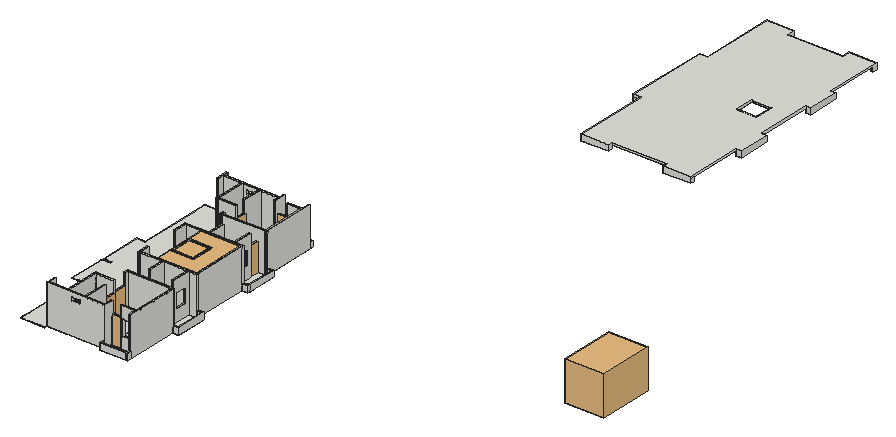
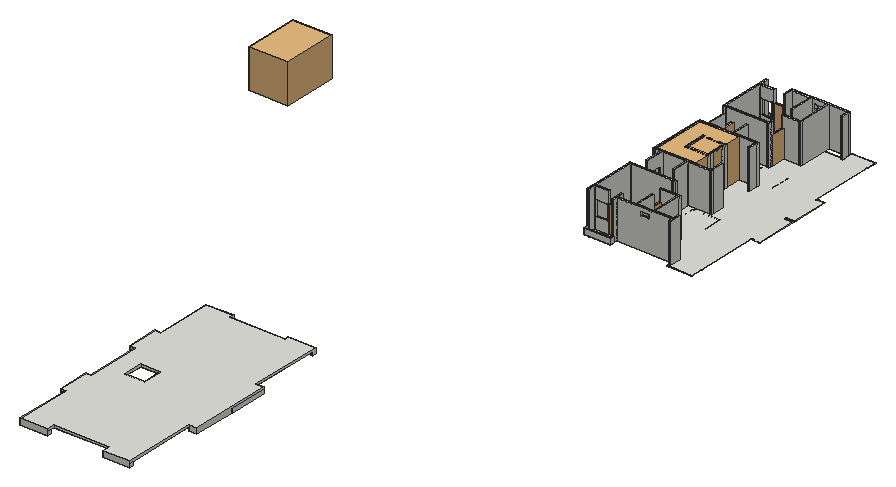
# SketchUp Ruby script. Lengths in inches.
U = 1.inch
M = Sketchup.active_model
def pt(a) = Geom::Point3d.new(a.map { |v| v * U })
def face(e, loops, mat)
  f = e.add_face(loops[0].map { |a| pt(a) })
  loops[1..].each { |l| e.add_face(l.map { |a| pt(a) }).erase! }
  f.material = f.back_material = mat if mat
  f
end
# faces: each face lists its corners as indices into pts; further lists are holes
def faces(e, pts, list, mat = nil) = list.each { |f| face(e, (f[0].is_a?(Array) ? f : [f]).map { |l| l.map { |i| pts[i] } }, mat) }
# xy, xz, yz: faces in a plane at the given z, y or x. An outline is a flat list of corners, or four numbers for a rectangle; further outlines are holes
def ring(l) = l.size == 4 ? [[l[0], l[1]], [l[2], l[1]], [l[2], l[3]], [l[0], l[3]]] : l.each_slice(2).to_a
def flat(e, list, mat, &to3) = list.each { |f| face(e, (f[0].is_a?(Array) ? f : [f]).map { |l| ring(l).map { |u, v| to3.(u, v) } }, mat) }
def xy(e, z, list, mat = nil) = flat(e, list, mat) { |x, y| [x, y, z] }
def xz(e, y, list, mat = nil) = flat(e, list, mat) { |x, z| [x, y, z] }
def yz(e, x, list, mat = nil) = flat(e, list, mat) { |y, z| [x, y, z] }
def lines(e, pts, list) = list.each { |a, b| e.add_line(pt(pts[a]), pt(pts[b])) }
# prism: a flat outline (further loops are holes) pulled along v
def prism(e, loops, v, mat = nil)
  f = face(e, loops, mat); d = Geom::Vector3d.new(v.map { |x| x * U })
  f.pushpull(f.normal.samedirection?(d) ? d.length : -d.length)
end
def box(e, o, s, mat = nil) = prism(e, [[o, [o[0] + s[0], o[1], o[2]], [o[0] + s[0], o[1] + s[1], o[2]], [o[0], o[1] + s[1], o[2]]]], [0, 0, s[2]], mat)
def at(x, y, z, deg = 0) = Geom::Transformation.translation(pt([x, y, z])) * Geom::Transformation.rotation(ORIGIN, Z_AXIS, deg.degrees)
def axes(o, x, y, z) = Geom::Transformation.new([*x, 0, *y, 0, *z, 0, *pt(o).to_a, 1])
def part(name) = M.definitions.add(name)
# library, detail: a bought-in or finely detailed component or shape, given as its bounding box
def library(name, o, s) = part(name).tap { |d| box(d.entities, o, s) }
def detail(e, o, s) = box(e.add_group.entities, o, s)
def put(e, d, t, mat = nil) = e.add_instance(d, t).tap { |i| i.material = mat if mat }
def group(e, t, mat = nil) = e.add_group.tap { |g| g.transformation = t; g.material = mat if mat }.entities
root = M.entities
M.materials.add("0-SS4").color = [255, 255, 255]
M.materials.add("0-SS7").color = [192, 192, 192]
M.materials.add("0-grey 3").color = [204, 204, 204]
M.materials.add("M09_Shadow_Night").color = [0, 0, 0]
c1 = part("Group\#84")
xy(c1.entities,0,[[[-2,-32,-2,-24,0.04,-24,0.04,0,0,0,0,198,-6,198,-6,196,-25.9,196,-25.9,312.57,0,312.57,0,318.21,-25.9,318.21,-25.9,446,-6,446,-6,444,0,444,0,675.78,72,673.93,76,673.93,76,665.93,74,665.93,74,636,252.4,636,252.4,673.93,328.4,673.93,328.4,636,324.4,636,324.4,498.14,330.4,498.14,330.4,499.84,344.35,499.84,344.35,411,324.4,411,324.4,231,344.35,231,344.35,142,324.4,142,324.4,0,324.58,0,324.58,-24,326.4,-24,326.4,-32,250.4,-32,250.4,-24,252.4,-24,252.4,0,188.4,0,188.4,-18,140,-18,140,0,72,0,72,-24,74,-24,74,-32],[210.4,291,270.4,351]]])
xy(c1.entities,1,[[[-2,-32,74,-32,74,-24,72,-24,72,0,140,0,140,-18,188.4,-18,188.4,0,252.4,0,252.4,-24,250.4,-24,250.4,-32,326.4,-32,326.4,-24,324.58,-24,324.58,0,324.4,0,324.4,142,344.35,142,344.35,231,324.4,231,324.4,411,344.35,411,344.35,499.84,330.4,499.84,330.4,498.14,324.4,498.14,324.4,636,328.4,636,328.4,673.93,252.4,673.93,252.4,636,74,636,74,665.93,76,665.93,76,673.93,72,673.93,0,675.78,0,444,-6,444,-6,446,-25.9,446,-25.9,318.21,0,318.21,0,312.57,-25.9,312.57,-25.9,196,-6,196,-6,198,0,198,0,0,0.04,0,0.04,-24,-2,-24],[210.4,291,270.4,351]]])
xz(c1.entities,-32,[[-2,0,74,1],[250.4,0,326.4,1]])
xz(c1.entities,-24,[[-2,0,0.04,1],[72,0,74,1],[250.4,0,252.4,1],[324.58,0,326.4,1]])
xz(c1.entities,-18,[[140,0,188.4,1]])
xz(c1.entities,0,[[0,0,0.04,1],[72,0,140,1],[188.4,0,252.4,1],[324.4,0,324.58,1]])
xz(c1.entities,142,[[324.4,0,344.35,1]])
xz(c1.entities,196,[[-25.9,0,-6,1]])
xz(c1.entities,198,[[-6,0,0,1]])
xz(c1.entities,231,[[324.4,0,344.35,1]])
xz(c1.entities,291,[[210.4,0,270.4,1]])
xz(c1.entities,312.57,[[-25.9,0,0,1]])
xz(c1.entities,318.21,[[-25.9,0,0,1]])
xz(c1.entities,351,[[210.4,0,270.4,1]])
xz(c1.entities,411,[[324.4,0,344.35,1]])
xz(c1.entities,444,[[-6,0,0,1]])
xz(c1.entities,446,[[-25.9,0,-6,1]])
xz(c1.entities,498.14,[[324.4,0,330.4,1]])
xz(c1.entities,499.84,[[330.4,0,344.35,1]])
xz(c1.entities,636,[[74,0,252.4,1],[324.4,0,328.4,1]])
xz(c1.entities,665.93,[[74,0,76,1]])
xz(c1.entities,673.93,[[72,0,76,1],[252.4,0,328.4,1]])
yz(c1.entities,-25.9,[[196,0,312.57,1],[318.21,0,446,1]])
yz(c1.entities,-6,[[196,0,198,1],[444,0,446,1]])
yz(c1.entities,-2,[[-32,0,-24,1]])
yz(c1.entities,0,[[0,0,198,1],[312.57,0,318.21,1],[444,0,636,1],[636,0,637.85,1],[637.85,0,675.78,1]])
yz(c1.entities,0.04,[[-24,0,0,1]])
yz(c1.entities,72,[[-24,0,0,1]])
yz(c1.entities,74,[[-32,0,-24,1],[636,0,665.93,1]])
yz(c1.entities,76,[[665.93,0,673.93,1]])
yz(c1.entities,140,[[-18,0,0,1]])
yz(c1.entities,188.4,[[-18,0,0,1]])
yz(c1.entities,210.4,[[291,0,351,1]])
yz(c1.entities,250.4,[[-32,0,-24,1]])
yz(c1.entities,252.4,[[-24,0,0,1],[636,0,673.93,1]])
yz(c1.entities,270.4,[[291,0,351,1]])
yz(c1.entities,324.4,[[0,0,142,1],[231,0,411,1],[498.14,0,636,1]])
yz(c1.entities,324.58,[[-24,0,0,1]])
yz(c1.entities,326.4,[[-32,0,-24,1]])
yz(c1.entities,328.4,[[636,0,673.93,1]])
yz(c1.entities,330.4,[[498.14,0,499.84,1]])
yz(c1.entities,344.35,[[142,0,231,1],[411,0,499.84,1]])
# 3 loose lines left out
p = [[77.67,648,0],[77.67,636,1],[246.4,636,1],[246.4,648,0],[72,673.93,0],[0,675.78,0],
  [0,675.78,1],[72,673.93,1]]
faces(c1.entities,p,[[0,1,2,3],[4,5,6,7]])
c2 = library("A$C72E23588",[-1177.7,-903.95,0],[2355.4,1807.9,0.01])
c3 = library("ghgjg",[-265.23,-341.01,0],[530.46,682.02,0.01])
c4 = part("Group\#15")
xy(c4.entities,0,[[60,-108.67,66,-102.67],[66,-108.67,120.4,-102.67],[60,-102.67,66,-12.67],[114.4,-72.67,120.4,-12.67],[0,-30.67,6,-12.67],
  [174.4,-30.67,180.4,-12.67],[0,-12.67,6,-6.67],[6,-12.67,60,-6.67],[60,-12.67,66,-6.67],[66,-12.67,114.4,-6.67],
  [114.4,-12.67,120.4,-6.67],[120.4,-12.67,174.4,-6.67],[174.4,-12.67,180.4,-6.67],[0,-6.67,6,0],[174.4,-6.67,180.4,5.26],
  [0,0,6,5.26]])
xy(c4.entities,96,[[78,-12.67,102.4,-6.67]])
xy(c4.entities,108,[[78,-12.67,102.4,-6.67]])
xy(c4.entities,120,[[60,-108.67,66,-102.67],[66,-108.67,120.4,-102.67],[60,-102.67,66,-12.67],[114.4,-72.67,120.4,-12.67],[0,-30.67,6,-12.67],
  [174.4,-30.67,180.4,-12.67],[0,-12.67,6,-6.67],[6,-12.67,60,-6.67],[60,-12.67,66,-6.67],[66,-12.67,114.4,-6.67],
  [114.4,-12.67,120.4,-6.67],[120.4,-12.67,174.4,-6.67],[174.4,-12.67,180.4,-6.67],[0,-6.67,6,0],[174.4,-6.67,180.4,5.26],
  [0,0,6,5.26]])
xz(c4.entities,-108.67,[[60,0,66,120],[66,0,120.4,120]])
xz(c4.entities,-102.67,[[60,0,66,120],[66,0,120.4,120]])
xz(c4.entities,-72.67,[[114.4,0,120.4,120]])
xz(c4.entities,-30.67,[[0,0,6,120],[174.4,0,180.4,120]])
xz(c4.entities,-12.67,[[6,0,60,120],[60,0,66,120],[[66,0,114.4,120],[78,96,102.4,108]],[114.4,0,120.4,120],[120.4,0,174.4,120]])
xz(c4.entities,-6.67,[[[6,0,174.4,120],[78,96,102.4,108]]])
xz(c4.entities,5.26,[[0,0,6,120],[174.4,0,180.4,120]])
yz(c4.entities,0,[[-30.67,0,5.26,120]])
yz(c4.entities,6,[[-30.67,0,-12.67,120],[-12.67,0,-6.67,120],[-6.67,0,0,120],[0,0,5.26,120]])
yz(c4.entities,60,[[-108.67,0,-102.67,120],[-102.67,0,-12.67,120]])
yz(c4.entities,66,[[-108.67,0,-102.67,120],[-102.67,0,-12.67,120]])
yz(c4.entities,78,[[-12.67,96,-6.67,108]])
yz(c4.entities,102.4,[[-12.67,96,-6.67,108]])
yz(c4.entities,114.4,[[-72.67,0,-12.67,120]])
yz(c4.entities,120.4,[[-108.67,0,-102.67,120],[-72.67,0,-12.67,120]])
yz(c4.entities,174.4,[[-30.67,0,-12.67,120],[-12.67,0,-6.67,120],[-6.67,0,5.26,120]])
yz(c4.entities,180.4,[[-30.67,0,5.26,120]])
c5 = part("tgr")
p = [[-2.37,-3.35,0],[-2.37,-2.82,0],[-2.73,-2.82,0],[-2.73,-2.68,0],[-3.71,-2.68,0],[-3.71,-3.35,0],
  [-2.37,3.35,0],[-2.37,2.82,0],[-2.73,2.82,0],[-2.73,2.68,0],[-3.71,2.68,0],[-3.71,3.35,0],
  [3.71,-2.82,0],[-2.37,-2.46,0],[3.71,-2.46,0],[3.7,-2.46,0],[3.63,-2.07,0],[3.53,-1.68,0],
  [3.41,-1.3,0],[3.27,-0.93,0],[3.1,-0.57,0],[2.91,-0.22,0],[2.7,0.12,0],[2.46,0.4375,0],
  [2.21,0.74,0],[1.93,1.03,0],[1.64,1.3,0],[1.33,1.55,0],[1.01,1.79,0],[0.67,1.99,0],
  [0.32,2.18,0],[-0.04,2.35,0],[-0.41,2.49,0],[-0.8,2.6,0],[-1.18,2.69,0],[-1.58,2.76,0],
  [-1.97,2.8,0]]
lines(c5.entities,p,[[0,1],[1,2],[2,3],[3,4],[4,5],[5,0],[6,7],[7,8],[8,9],[9,10],[10,11],[11,6],
  [1,12],[13,14],[1,13],[12,14],[15,16],[16,17],[17,18],[18,19],[19,20],[20,21],[21,22],[22,23],
  [23,24],[24,25],[25,26],[26,27],[27,28],[28,29],[29,30],[30,31],[31,32],[32,33],[33,34],[34,35],
  [35,36],[36,7]])
c6 = library("Group\#49",[0,0,0],[8.31,30,84])
c7 = library("Group\#50",[0,0,0],[6.9375,42,86.5])
c8 = library("Group\#51",[0,0,0],[6.9375,42,86.5])
c9 = part("G5GTGTGT")
p = [[0.52,4.97,0],[0.52,-4.97,0],[0.36,-4.97,0],[0.36,4.97,0],[-0.08,-4.53,0],[-0.08,4.53,0],
  [0.33,4.97,0],[0.3,4.97,0],[0.28,4.96,0],[0.25,4.96,0],[0.22,4.95,0],[0.2,4.94,0],
  [0.17,4.93,0],[0.15,4.92,0],[0.12,4.9,0],[0.1,4.89,0],[0.08,4.87,0],[0.06,4.85,0],
  [0.04,4.83,0],[0.02,4.8125,0],[0,4.79,0],[-0.01,4.77,0],[-0.03,4.74,0],[-0.04,4.72,0],
  [-0.05,4.69,0],[-0.0625,4.67,0],[-0.07,4.64,0],[-0.08,4.61,0],[-0.08,4.59,0],[-0.08,4.56,0],
  [-0.08,-4.56,0],[-0.08,-4.59,0],[-0.08,-4.61,0],[-0.07,-4.64,0],[-0.0625,-4.67,0],[-0.05,-4.69,0],
  [-0.04,-4.72,0],[-0.03,-4.74,0],[-0.01,-4.77,0],[0,-4.79,0],[0.02,-4.8125,0],[0.04,-4.83,0],
  [0.06,-4.85,0],[0.08,-4.87,0],[0.1,-4.89,0],[0.12,-4.9,0],[0.15,-4.92,0],[0.17,-4.93,0],
  [0.2,-4.94,0],[0.22,-4.95,0],[0.25,-4.96,0],[0.28,-4.96,0],[0.3,-4.97,0],[0.33,-4.97,0],
  [-0.08,-1.38,0],[-0.52,-1.38,0],[-0.08,1.38,0],[-0.52,1.38,0]]
lines(c9.entities,p,[[0,1],[1,2],[2,3],[3,0],[4,5],[3,6],[6,7],[7,8],[8,9],[9,10],[10,11],[11,12],
  [12,13],[13,14],[14,15],[15,16],[16,17],[17,18],[18,19],[19,20],[20,21],[21,22],[22,23],[23,24],
  [24,25],[25,26],[26,27],[27,28],[28,29],[29,5],[4,30],[30,31],[31,32],[32,33],[33,34],[34,35],
  [35,36],[36,37],[37,38],[38,39],[39,40],[40,41],[41,42],[42,43],[43,44],[44,45],[45,46],[46,47],
  [47,48],[48,49],[49,50],[50,51],[51,52],[52,53],[53,2],[54,55],[56,57],[55,57]])
c10 = part("Lift Door")
g1 = group(c10.entities,at(22.98,-1.97,0))
xy(g1,0,[[-11.49,0,22.98,1.97]],"0-SS7")
xy(g1,81.69,[[-11.49,0,22.98,1.97]],"0-SS7")
xz(g1,0,[[-11.49,0,22.98,81.69]],"0-SS7")
xz(g1,1.97,[[-11.49,0,22.98,81.69]],"0-SS4")
yz(g1,-11.49,[[0,0,1.97,81.69]],"0-SS7")
yz(g1,22.98,[[0,0,1.97,81.69]],"0-SS7")
c11 = part("Group\#83")
put(c11.entities,c10,axes([5.4,10.39,0],[0,0.42899,0],[-0.53123,0,0],[0,0,1.07229]),"0-grey 3")
put(c11.entities,c10,axes([5.4,-4.4,0],[0,0.42899,0],[-0.53123,0,0],[0,0,1.07229]),"0-grey 3")
g2 = group(c11.entities,at(0,44.39,0))
p = [[0,-44.39,88.58],[0,-13.75,88.58],[0,-13.75,0],[0,-44.39,0]]
lines(g2,p,[[0,1],[1,2],[3,0],[2,3]])
g3 = group(c11.entities,at(2.42,30.63,0))
prism(g3,[[[2.98,-30.63,0],[2.98,-30.11,0],[2.98,-30.11,87.6],[2.98,-0.53,87.6],[2.98,-0.53,0],[2.98,0,0],[2.98,0,88.58],[2.98,-30.63,88.58]]],[-5.4,0,0])
c12 = part("EGWF")
p = [[2.59,-3.49,0],[2.59,-3.09,0],[2.85,-3.09,0],[2.85,-2.99,0],[3.58,-2.99,0],[3.58,-3.49,0],
  [2.59,3.49,0],[2.59,3.09,0],[2.85,3.09,0],[2.85,2.99,0],[3.58,2.99,0],[3.58,3.49,0],
  [-3.58,-3.09,0],[2.59,-2.82,0],[-3.58,-2.82,0],[2.2,3.07,0],[1.81,3.04,0],[1.42,2.97,0],
  [1.03,2.89,0],[0.66,2.78,0],[0.29,2.64,0],[-0.07,2.48,0],[-0.42,2.3,0],[-0.76,2.1,0],
  [-1.08,1.875,0],[-1.39,1.63,0],[-1.68,1.37,0],[-1.96,1.09,0],[-2.21,0.79,0],[-2.45,0.48,0],
  [-2.67,0.15,0],[-2.86,-0.1875,0],[-3.04,-0.54,0],[-3.1875,-0.9,0],[-3.32,-1.28,0],[-3.42,-1.66,0],
  [-3.5,-2.04,0],[-3.55,-2.43,0]]
lines(c12.entities,p,[[0,1],[1,2],[2,3],[3,4],[4,5],[5,0],[6,7],[7,8],[8,9],[9,10],[10,11],[11,6],
  [1,12],[13,14],[1,13],[12,14],[7,15],[15,16],[16,17],[17,18],[18,19],[19,20],[20,21],[21,22],
  [22,23],[23,24],[24,25],[25,26],[26,27],[27,28],[28,29],[29,30],[30,31],[31,32],[32,33],[33,34],
  [34,35],[35,36],[36,37],[37,14]])
c13 = library("Component\#2",[1075.72,38.58,0],[54,24,0.01])
c14 = library("Component\#4",[1075.72,686.58,0],[54,18,0.01])
c15 = part("Group\#53")
xy(c15.entities,0,[[-66,-66,-60,-60],[-60,-66,0,-60],[0,-66,6,-60],[-66,-60,-60,-48.73],[0,-60,6,0],
  [-66,-12.73,-60,0],[-66,0,-60,6],[-60,0,0,6],[0,0,6,6]])
xy(c15.entities,120,[[-66,-66,-60,-60],[-60,-66,0,-60],[0,-66,6,-60],[-66,-60,-60,-48.73],[0,-60,6,0],
  [-66,-12.73,-60,0],[-66,0,-60,6],[-60,0,0,6],[0,0,6,6]])
xz(c15.entities,-66,[[-66,0,-60,120],[-60,0,0,120],[0,0,6,120]])
xz(c15.entities,-60,[[-66,0,-60,120],[-60,0,0,120],[0,0,6,120]])
xz(c15.entities,-48.73,[[-66,0,-60,120]])
xz(c15.entities,-12.73,[[-66,0,-60,120]])
xz(c15.entities,0,[[-66,0,-60,120],[-60,0,0,120],[0,0,6,120]])
xz(c15.entities,6,[[-66,0,-60,120],[-60,0,0,120],[0,0,6,120]])
yz(c15.entities,-66,[[-66,0,-60,120],[-60,0,-48.73,120],[-12.73,0,0,120],[0,0,6,120]])
yz(c15.entities,-60,[[-66,0,-60,120],[-60,0,-48.73,120],[-12.73,0,0,120],[0,0,6,120]])
yz(c15.entities,0,[[-66,0,-60,120],[-60,0,0,120],[0,0,6,120]])
yz(c15.entities,6,[[-66,0,-60,120],[-60,0,0,120],[0,0,6,120]])
c16 = part("Group\#12")
xy(c16.entities,0,[[0,0,6,7.18],[0,7.18,6,168],[-174.4,129.21,-168.4,168],[-174.4,168,-168.4,174],[-168.4,168,-102,174],
  [-102,168,-96,174],[-96,168,0,174],[0,168,6,174],[6,168,24,174],[-102,174,-96,225]])
xy(c16.entities,18,[[6,168,24,174]],"M09_Shadow_Night")
xy(c16.entities,120,[[0,0,6,7.18],[0,7.18,6,168],[-174.4,129.21,-168.4,168],[-174.4,168,-168.4,174],[-168.4,168,-102,174],
  [-102,168,-96,174],[-96,168,0,174],[0,168,6,174],[-102,174,-96,225]])
xz(c16.entities,0,[[0,0,6,120]])
xz(c16.entities,129.21,[[-174.4,0,-168.4,120]])
xz(c16.entities,168,[[-174.4,0,-168.4,120],[-168.4,0,-102,120],[-102,0,-96,120],[-96,0,0,120],[0,0,6,120],
  [6,0,24,18]])
xz(c16.entities,174,[[-174.4,0,-168.4,120],[-168.4,0,-102,120],[-102,0,-96,120],[-96,0,0,120],[0,0,6,120],
  [6,0,24,18]])
xz(c16.entities,225,[[-102,0,-96,120]])
yz(c16.entities,-174.4,[[129.21,0,168,120],[168,0,174,120]])
yz(c16.entities,-168.4,[[129.21,0,168,120],[168,0,174,120]])
yz(c16.entities,-102,[[168,0,174,120],[174,0,225,120]])
yz(c16.entities,-96,[[168,0,174,120],[174,0,225,120]])
yz(c16.entities,0,[[0,0,7.18,120],[7.18,0,168,120],[168,0,174,120]])
yz(c16.entities,6,[[0,0,168,120],[168,0,174,18],[168,18,174,120]])
yz(c16.entities,24,[[168,0,174,18]])
c17 = part("Group\#11")
xy(c17.entities,0,[[0,0,5.15,4],[5.15,0,13.95,4],[13.95,0,18,4],[13.95,4,18,93],[-30,36,-24,93],
  [-108,42,-102,93],[-180.4,93,-174.4,99],[-174.4,93,-108,99],[-108,93,-102,99],[-102,93,-24,99],
  [-24,93,-6,99],[-6,93,0,99],[0,93,13.95,99],[13.95,93,18,99],[-180.4,99,-174.4,126.21]])
xy(c17.entities,20,[[0,0,18,4],[13.95,4,18,4,18,99,0,99,0,93,13.95,93]],"M09_Shadow_Night")
xy(c17.entities,36,[[-30,42,-24,81]])
xy(c17.entities,84,[[-30,42,-24,81]])
xy(c17.entities,120,[[-30,36,-24,93],[-108,42,-102,93],[-180.4,93,-174.4,99],[-174.4,93,-108,99],[-108,93,-102,99],
  [-102,93,-24,99],[-24,93,0,99],[-180.4,99,-174.4,126.21]])
xz(c17.entities,0,[[0,0,18,20]])
xz(c17.entities,4,[[0,0,5.15,20],[5.15,0,13.95,20]])
xz(c17.entities,36,[[-30,0,-24,120]])
xz(c17.entities,42,[[-108,0,-102,120],[-30,36,-24,84]])
xz(c17.entities,81,[[-30,36,-24,84]])
xz(c17.entities,93,[[-180.4,0,-174.4,120],[-174.4,0,-108,120],[-108,0,-102,120],[-102,0,-30,120],[-30,0,-24,120],
  [-24,0,0,120],[0,0,13.95,20]])
xz(c17.entities,99,[[-180.4,0,-174.4,120],[-174.4,0,-108,120],[-108,0,-102,120],[-102,0,-24,120],[-24,0,-6,120],
  [-6,0,0,120],[0,0,18,20]])
xz(c17.entities,126.21,[[-180.4,0,-174.4,120]])
yz(c17.entities,-180.4,[[93,0,99,120],[99,0,126.21,120]])
yz(c17.entities,-174.4,[[93,0,99,120],[99,0,126.21,120]])
yz(c17.entities,-108,[[42,0,93,120],[93,0,99,120]])
yz(c17.entities,-102,[[42,0,93,120],[93,0,99,120]])
yz(c17.entities,-30,[[[36,0,93,120],[42,36,81,84]]])
yz(c17.entities,-24,[[[36,0,93,120],[42,36,81,84]],[93,0,99,120]])
yz(c17.entities,0,[[0,0,4,20],[93,0,99,20],[93,20,99,120]])
yz(c17.entities,13.95,[[4,0,93,20]])
yz(c17.entities,18,[[0,0,99,20]])
c18 = library("burner",[-300,-225,0],[600,450,0.01])
c19 = part("Group\#10")
xy(c19.entities,0,[[-133.3,-6,-127.3,0],[-133.3,0,-127.3,6],[-127.3,0,0,6],[0,0,10.7,6]])
xy(c19.entities,120,[[-133.3,-6,-127.3,0],[-133.3,0,-127.3,6],[-127.3,0,0,6],[0,0,10.7,6]])
xz(c19.entities,-6,[[-133.3,0,-127.3,120]])
xz(c19.entities,0,[[-133.3,0,-127.3,120],[-127.3,0,0,120],[0,0,10.7,120]])
xz(c19.entities,6,[[-133.3,0,-127.3,120],[-127.3,0,0,120],[0,0,10.7,120]])
yz(c19.entities,-133.3,[[-6,0,0,120],[0,0,6,120]])
yz(c19.entities,-127.3,[[-6,0,0,120],[0,0,6,120]])
yz(c19.entities,0,[[0,0,6,120]])
yz(c19.entities,10.7,[[0,0,6,120]])
c20 = part("Group\#126")
xy(c20.entities,0,[[-138,-162.42,-132,-156.42],[-132,-162.42,0,-156.42],[0,-162.42,6,-156.42],[-138,-156.42,-132,-150.42],[0,-156.42,6,-24.42],
  [-42,-24.42,0,-18.42],[0,-24.42,6,-18.42],[0,-18.42,6,0],[0,0,6,5.51]])
xy(c20.entities,36,[[-40,-24.42,-2,-18.42]])
xy(c20.entities,84,[[-40,-24.42,-2,-18.42]])
xy(c20.entities,120,[[-138,-162.42,-132,-156.42],[-132,-162.42,0,-156.42],[0,-162.42,6,-156.42],[-138,-156.42,-132,-150.42],[0,-156.42,6,-24.42],
  [-42,-24.42,0,-18.42],[0,-24.42,6,-18.42],[0,-18.42,6,0],[0,0,6,5.51]])
xz(c20.entities,-162.42,[[-138,0,-132,120],[-132,0,0,120],[0,0,6,120]])
xz(c20.entities,-156.42,[[-138,0,-132,120],[-132,0,0,120],[0,0,6,120]])
xz(c20.entities,-150.42,[[-138,0,-132,120]])
xz(c20.entities,-24.42,[[[-42,0,0,120],[-40,36,-2,84]]])
xz(c20.entities,-18.42,[[[-42,0,0,120],[-40,36,-2,84]]])
xz(c20.entities,5.51,[[0,0,6,120]])
yz(c20.entities,-138,[[-162.42,0,-156.42,120],[-156.42,0,-150.42,120]])
yz(c20.entities,-132,[[-162.42,0,-156.42,120],[-156.42,0,-150.42,120]])
yz(c20.entities,-42,[[-24.42,0,-18.42,120]])
yz(c20.entities,-40,[[-24.42,36,-18.42,84]])
yz(c20.entities,-2,[[-24.42,36,-18.42,84]])
yz(c20.entities,0,[[-162.42,0,-156.42,120],[-156.42,0,-24.42,120],[-24.42,0,-18.42,120],[-18.42,0,0,120],[0,0,5.51,120]])
yz(c20.entities,6,[[-162.42,0,-156.42,120],[-156.42,0,5.51,120]])
c21 = library("Return staircase",[0,-11.89,0],[120,168,120])
c22 = part("Component\#5")
p = [[1166.02,522.1,0],[1167.27,522.1,0],[1183.11,522.1,0],[1183.72,522.1,0],[1165.72,517.1,0],[1167.27,517.1,0],
  [1183.11,517.1,0],[1183.72,517.1,0],[1165.72,512.1,0],[1167.27,512.1,0],[1183.11,512.1,0],[1183.72,512.1,0],
  [1165.72,507.1,0],[1167.27,507.1,0],[1183.11,507.1,0],[1183.72,507.1,0],[1165.72,502.1,0],[1167.27,502.1,0],
  [1183.11,502.1,0],[1183.72,502.1,0],[1165.72,497.1,0],[1167.27,497.1,0],[1183.11,497.1,0],[1183.72,497.1,0],
  [1165.72,492.1,0],[1183.72,492.1,0],[1165.72,487.1,0],[1183.72,487.1,0],[1111.72,482.1,0],[1128.65,482.1,0],
  [1150.05,482.1,0],[1183.72,482.1,0],[1111.72,477.1,0],[1128.65,477.1,0],[1150.05,477.1,0],[1183.72,477.1,0],
  [1111.72,472.1,0],[1128.65,472.1,0],[1150.05,472.1,0],[1173.72,472.1,0],[1117.28,469.6,0],[1112.28,474.6,0],
  [1127.28,479.6,0],[1122.28,484.6,0],[1157.28,469.6,0],[1152.28,474.6,0],[1173.72,473.16,0],[1172.28,474.6,0],
  [1167.28,479.6,0],[1162.28,484.6,0],[1183.72,483.16,0],[1182.28,484.6,0],[1177.28,489.6,0],[1172.48,494.4,0],
  [1167.27,499.61,0],[1165.72,501.16,0],[1183.72,503.16,0],[1183.11,503.77,0],[1167.27,519.61,0],[1165.77,521.11,0],
  [1183.72,523.16,0],[1182.3,524.58,0],[1118.53,469.6,0],[1113.53,474.6,0],[1128.53,479.6,0],[1123.53,484.6,0],
  [1158.53,469.6,0],[1153.53,474.6,0],[1173.72,474.41,0],[1173.53,474.6,0],[1168.53,479.6,0],[1163.53,484.6,0],
  [1183.72,484.41,0],[1183.53,484.6,0],[1178.53,489.6,0],[1173.73,494.4,0],[1167.27,500.86,0],[1165.72,502.41,0],
  [1183.72,504.41,0],[1183.53,504.6,0],[1167.27,520.86,0],[1166.02,522.11,0],[1183.72,524.41,0],[1183.55,524.58,0],
  [1119.78,469.6,0],[1114.78,474.6,0],[1128.65,480.73,0],[1124.78,484.6,0],[1159.78,469.6,0],[1154.78,474.6,0],
  [1169.78,479.6,0],[1164.78,484.6,0],[1179.78,489.6,0],[1174.98,494.4,0],[1167.27,502.11,0],[1165.72,503.66,0],
  [1167.27,522.11,0],[1166.48,522.9,0]]
lines(c22.entities,p,[[0,1],[2,3],[4,5],[6,7],[8,9],[10,11],[12,13],[14,15],[16,17],[18,19],[20,21],[22,23],
  [24,25],[26,27],[28,29],[30,31],[32,33],[34,35],[36,37],[38,39],[40,41],[42,43],[44,45],[46,47],
  [48,49],[50,51],[52,53],[54,55],[56,57],[58,59],[60,61],[62,63],[64,65],[66,67],[68,69],[70,71],
  [72,73],[74,75],[76,77],[78,79],[80,81],[82,83],[84,85],[86,87],[88,89],[90,91],[92,93],[94,95],
  [96,97]])
c23 = library("Group\#48",[0,0,0],[6.9375,42,86.5])
c24 = library("double bed",[-999.9375,-1062.5,0],[1999.875,2125,0.01])
c25 = part("Group\#8")
xy(c25.entities,0,[[0,-8.88,4,-4.88],[4,-8.88,80,-4.88],[80,-8.88,84,-4.88],[0,-4.88,4,0],[80,-4.88,84,3.12],
  [0,0,4,3.12]])
xy(c25.entities,20,[[0,-8.88,4,-4.88],[4,-8.88,80,-4.88],[80,-8.88,84,-4.88],[0,-4.88,4,0],[80,-4.88,84,3.12],
  [0,0,4,3.12]],"M09_Shadow_Night")
xz(c25.entities,-8.88,[[0,0,80,20],[80,0,84,20]])
xz(c25.entities,-4.88,[[4,0,80,20]])
xz(c25.entities,3.12,[[0,0,4,20],[80,0,84,20]])
yz(c25.entities,0,[[-8.88,0,3.12,20]])
yz(c25.entities,4,[[-4.88,0,0,20],[0,0,3.12,20]])
yz(c25.entities,80,[[-8.88,0,-4.88,20],[-4.88,0,3.12,20]])
yz(c25.entities,84,[[-8.88,0,3.12,20]])
c26 = part("Group\#16")
xy(c26.entities,0,[[0,0,4,3.74],[80,0,84,8],[0,3.74,4,8],[0,8,4,12],[4,8,80,12],
  [80,8,84,12]])
xy(c26.entities,18,[[0,0,4,12],[80,0,84,0,84,12,4,12,4,8,80,8]],"M09_Shadow_Night")
xz(c26.entities,0,[[0,0,4,18],[80,0,84,18]])
xz(c26.entities,8,[[4,0,80,18]])
xz(c26.entities,12,[[0,0,84,18]])
yz(c26.entities,0,[[0,0,12,18]])
yz(c26.entities,4,[[0,0,3.74,18],[3.74,0,8,18]])
yz(c26.entities,80,[[0,0,8,18]])
yz(c26.entities,84,[[0,0,12,18]])
c27 = library("sink",[-449.92,-250,0],[899.84,500,0.01])
c28 = part("GTGTGYHYHYHY")
p = [[-3.29,3.76,0],[3.29,3.76,0],[3.29,-3.76,0],[-3.29,-3.76,0]]
lines(c28.entities,p,[[0,1],[1,2],[2,3],[3,0],[0,2],[1,3]])
c29 = library("TREE-26",[-60.96,-72.91,0],[121.92,134.74,0.01])
c30 = part("Group\#14")
xy(c30.entities,0,[[0,0,4.05,3.45],[0,3.45,4.05,88.84],[-13.95,88.84,0,93],[0,88.84,4.05,93]])
xy(c30.entities,18,[[0,0,4.05,88.84],[-13.95,88.84,0,93],[0,88.84,4.05,93]],"M09_Shadow_Night")
xz(c30.entities,0,[[0,0,4.05,18]])
xz(c30.entities,88.84,[[-13.95,0,0,18]])
xz(c30.entities,93,[[-13.95,0,4.05,18]])
yz(c30.entities,-13.95,[[88.84,0,93,18]])
yz(c30.entities,0,[[0,0,3.45,18],[3.45,0,88.84,18]])
yz(c30.entities,4.05,[[0,0,93,18]])
c31 = part("Group\#111")
xy(c31.entities,-36.67,[[252.4,-12,252.4,0,259.49,0,259.49,-8,330.4,-8,330.4,0,336.4,0,336.4,-12]])
xy(c31.entities,-36.53,[[0,-12,0,-0.08,6,-0.08,6,-8,78,-8,78,0,84,0,84,-12],[336.4,163,336.4,169,349.41,169,349.41,255,336.4,255,336.4,261,353.41,261,353.41,163],[-24,217,-24,336.57,-20,336.57,-20,222,0,222,0,217],[-24,342.21,-24,473,0,473,0,468,-20,468,-20,342.21],[336.4,430,336.4,435,347.875,435,347.875,523,335.62,523,335.62,528,351.875,528,351.875,430],
  [0,689.93,0,701.93,84,701.93,84,689.93,78,689.93,78,697.93,6,697.93,6,689.93],[252.4,689.93,252.4,701.93,336.4,701.93,336.4,689.93,330.4,689.93,330.4,697.93,258.4,697.93,258.4,689.93]])
xy(c31.entities,-24.53,[[[6,-8,6,-0.08,0,-0.08,0,222,-20,222,-20,336.57,-24,336.57,-24,342.21,-20,342.21,-20,468,0,468,0,689.93,6,689.93,6,697.93,78,697.93,78,689.93,84,689.93,84,678,252.4,678,252.4,689.93,258.4,689.93,258.4,697.93,330.4,697.93,330.4,689.93,336.4,689.93,336.4,528,335.62,528,335.62,523,347.875,523,347.875,435,336.4,435,336.4,255,349.41,255,349.41,169,336.4,169,336.4,0,330.4,0,330.4,-8,259.49,-8,259.49,0,78,0,78,-8],[216.4,315,276.4,375]],[-24,217,0,217,0,222,-20,222,-20,336.57,-24,336.57]])
xy(c31.entities,-18.53,[[[0,-12,84,-12,84,0,252.4,0,252.4,-12,336.4,-12,336.4,163,353.41,163,353.41,261,336.4,261,336.4,430,351.875,430,351.875,528,336.4,528,336.4,701.93,252.4,701.93,252.4,678,84,678,84,701.93,0,701.93,0,473,-24,473,-24,217,0,217],[216.4,315,276.4,375]]])
xz(c31.entities,-12,[[252.4,-36.67,336.4,-18.53],[0,-36.53,84,-18.53]])
xz(c31.entities,-8,[[259.49,-36.67,330.4,-24.53],[6,-36.53,78,-24.53]])
xz(c31.entities,-0.08,[[0,-36.53,6,-24.53]])
xz(c31.entities,0,[[252.4,-36.67,259.49,-24.53],[330.4,-36.67,336.4,-24.53],[78,-36.53,84,-24.53],[84,-24.53,252.4,-18.53]])
xz(c31.entities,163,[[336.4,-36.53,353.41,-18.53]])
xz(c31.entities,169,[[336.4,-36.53,349.41,-24.53]])
xz(c31.entities,217,[[-24,-36.53,0,-24.53],[-24,-24.53,0,-18.53]])
xz(c31.entities,222,[[-20,-36.53,0,-24.53]])
xz(c31.entities,255,[[336.4,-36.53,349.41,-24.53]])
xz(c31.entities,261,[[336.4,-36.53,353.41,-18.53]])
xz(c31.entities,315,[[216.4,-24.53,276.4,-18.53]])
xz(c31.entities,336.57,[[-24,-36.53,-20,-24.53]])
xz(c31.entities,342.21,[[-24,-36.53,-20,-24.53]])
xz(c31.entities,375,[[216.4,-24.53,276.4,-18.53]])
xz(c31.entities,430,[[336.4,-36.53,351.875,-18.53]])
xz(c31.entities,435,[[336.4,-36.53,347.875,-24.53]])
xz(c31.entities,468,[[-20,-36.53,0,-24.53]])
xz(c31.entities,473,[[-24,-36.53,0,-18.53]])
xz(c31.entities,523,[[335.62,-36.53,347.875,-24.53]])
xz(c31.entities,528,[[335.62,-36.53,351.875,-24.53],[336.4,-24.53,351.875,-18.53]])
xz(c31.entities,678,[[84,-24.53,252.4,-18.53]])
xz(c31.entities,689.93,[[0,-36.53,6,-24.53],[78,-36.53,84,-24.53],[252.4,-36.53,258.4,-24.53],[330.4,-36.53,336.4,-24.53]])
xz(c31.entities,697.93,[[6,-36.53,78,-24.53],[258.4,-36.53,330.4,-24.53]])
xz(c31.entities,701.93,[[0,-36.53,84,-18.53],[252.4,-36.53,336.4,-18.53]])
yz(c31.entities,-24,[[217,-36.53,336.57,-24.53],[342.21,-36.53,342.21,-24.53,217,-24.53,217,-18.53,473,-18.53,473,-36.53]])
yz(c31.entities,-20,[[222,-36.53,336.57,-24.53],[342.21,-36.53,468,-24.53]])
yz(c31.entities,0,[[-12,-36.53,-12,-18.53,217,-18.53,217,-24.53,-0.08,-24.53,-0.08,-36.53],[217,-36.53,222,-24.53],[468,-36.53,473,-24.53],[689.93,-36.53,701.93,-24.53],[473,-24.53,701.93,-18.53]])
yz(c31.entities,6,[[-8,-36.53,-0.08,-24.53],[689.93,-36.53,697.93,-24.53]])
yz(c31.entities,78,[[-8,-36.53,0,-24.53],[689.93,-36.53,697.93,-24.53]])
yz(c31.entities,84,[[-12,-36.53,0,-18.53],[689.93,-36.53,701.93,-36.53,701.93,-18.53,678,-18.53,678,-24.53,689.93,-24.53]])
yz(c31.entities,216.4,[[315,-24.53,375,-18.53]])
yz(c31.entities,252.4,[[-12,-36.67,0,-18.53],[689.93,-36.53,701.93,-24.53],[678,-24.53,701.93,-18.53]])
yz(c31.entities,258.4,[[689.93,-36.53,697.93,-24.53]])
yz(c31.entities,259.49,[[-8,-36.67,0,-24.53]])
yz(c31.entities,276.4,[[315,-24.53,375,-18.53]])
yz(c31.entities,330.4,[[-8,-36.67,0,-24.53],[689.93,-36.53,697.93,-24.53]])
yz(c31.entities,335.62,[[523,-36.53,528,-24.53]])
yz(c31.entities,336.4,[[-12,-36.67,0,-24.53],[163,-36.53,169,-24.53],[255,-36.53,261,-24.53],[430,-36.53,435,-24.53],[689.93,-36.53,701.93,-36.53,701.93,-18.53,528,-18.53,528,-24.53,689.93,-24.53],
  [-12,-24.53,163,-18.53],[261,-24.53,430,-18.53]])
yz(c31.entities,347.875,[[435,-36.53,523,-24.53]])
yz(c31.entities,349.41,[[169,-36.53,255,-24.53]])
yz(c31.entities,351.875,[[430,-36.53,528,-18.53]])
yz(c31.entities,353.41,[[163,-36.53,261,-18.53]])
box(root,[3822.86,1590.875,246],[54,18,1])
prism(root,[[[3936.86,1371.875,246],[3936.86,1428.875,246],[3936.86,1428.875,366],[3936.86,1371.875,366]],[[3936.86,1377.875,282],[3936.86,1377.875,330],[3936.86,1416.875,330],[3936.86,1416.875,282]]],[-6,0,0])
xy(root,246,[[3822.86,942.875,3876.86,966.64],[3816.86,1458.875,3960.86,1458.875,3960.86,1626.8,3954.86,1626.8,3954.86,1602.875,3912.86,1602.875,3912.86,1596.875,3954.86,1596.875,3954.86,1464.875,3822.86,1464.875,3822.86,1470.875,3816.86,1470.875]])
put(root,c1,at(3630.46,960.875,246))
put(root,c2,axes([3790.49,1151.05,246],[0.0356,0,0],[0,-0.0356,0],[0,0,0.0356]))
put(root,c2,axes([3790.49,1413,246],[0.0356,0,0],[0,-0.0356,0],[0,0,0.0356]))
put(root,c3,axes([3792.56,1595.13,246],[-0.04,0,0],[0,0.04,0],[0,0,0.04]))
put(root,c4,at(3702.46,1621.54,246))
g4 = group(root,at(3702.46,936.875,246))
xy(g4,0,[[0,0,6,6],[6,0,60,6],[60,0,66,6],[66,0,114.4,6],[114.4,0,120.4,6],
  [120.4,0,174.4,6],[174.4,0,180.4,6],[0,6,6,30],[60,6,66,108],[114.4,6,120.4,78],
  [174.4,6,180.4,30],[60,108,66,114],[66,108,120.4,114]])
xy(g4,96,[[78,0,102.4,6]])
xy(g4,108,[[78,0,102.4,6]])
xy(g4,120,[[0,0,6,6],[6,0,60,6],[60,0,66,6],[66,0,114.4,6],[114.4,0,120.4,6],
  [120.4,0,174.4,6],[174.4,0,180.4,6],[0,6,6,30],[60,6,66,108],[114.4,6,120.4,78],
  [174.4,6,180.4,30],[60,108,66,114],[66,108,120.4,114]])
xz(g4,0,[[[0,0,180.4,120],[78,96,102.4,108]]])
xz(g4,6,[[0,0,6,120],[6,0,60,120],[60,0,66,120],[[66,0,114.4,120],[78,96,102.4,108]],[114.4,0,120.4,120],
  [120.4,0,174.4,120]])
xz(g4,30,[[0,0,6,120],[174.4,0,180.4,120]])
xz(g4,78,[[114.4,0,120.4,120]])
xz(g4,108,[[60,0,66,120],[66,0,120.4,120]])
xz(g4,114,[[60,0,66,120],[66,0,120.4,120]])
yz(g4,0,[[0,0,6,120],[6,0,30,120]])
yz(g4,6,[[6,0,30,120]])
yz(g4,60,[[6,0,108,120],[108,0,114,120]])
yz(g4,66,[[6,0,108,120],[108,0,114,120]])
yz(g4,78,[[0,96,6,108]])
yz(g4,102.4,[[0,96,6,108]])
yz(g4,114.4,[[6,0,78,120]])
yz(g4,120.4,[[6,0,78,120],[108,0,114,120]])
yz(g4,174.4,[[6,0,30,120]])
yz(g4,180.4,[[0,0,30,120]])
put(root,c3,axes([3792.66,956.52,246],[0.04,0,0],[0,-0.04,0],[0,0,0.04]))
put(root,c5,axes([3806.26,1029.875,246],[-4.47464,0,0],[0,-4.47464,0],[0,0,4.47464]))
put(root,c5,axes([3806.26,1533.875,246],[-4.47464,0,0],[0,4.47464,0],[0,0,4.47464]))
put(root,c6,axes([3821.14,1512.875,246],[-1,0,0],[0,-1.4,0],[0,0,1]))
put(root,c7,axes([3815.2,1050.875,246],[0.85622,0,0],[0,1,0],[0,0,0.9711]))
put(root,c8,axes([3824.52,1548.875,246],[-0.85622,0,0],[0,-0.71429,0],[0,0,0.9711]))
put(root,c6,at(3818.58,1014.875,246))
put(root,c9,axes([3824.76,995.11,246],[3.62,0,0],[0,3.62,0],[0,0,3.62]))
put(root,c9,axes([3824.76,1569.29,246],[3.62,0,0],[0,3.62,0],[0,0,3.62]))
put(root,c11,axes([3834.86,1263.12,245.39],[1,0,0],[0,1.17593,0],[0,0,1.36155]))
put(root,c12,axes([3838.46,1491.875,246],[-6.02515,0,0],[0,6.02515,0],[0,0,6.02515]))
put(root,c12,axes([3838.46,1071.875,246],[-6.02515,0,0],[0,-6.02515,0],[0,0,6.02515]))
put(root,c13,at(2747.14,904.3,246))
put(root,c14,at(2747.14,904.3,246))
put(root,c15,at(3900.86,1311.875,246))
put(root,c16,at(3954.86,1197.875,246))
put(root,c17,at(3960.86,1098.875,246))
put(root,c18,axes([3886.49,1381.11,246],[-0.03566,0,0],[0,-0.03566,0],[0,0,0.03566]))
put(root,c19,at(3950.16,1098.875,246))
put(root,c20,at(3954.86,1621.3,246))
put(root,c21,at(3834.86,1209.77,246))
put(root,c22,at(2747.14,904.3,246))
put(root,c8,axes([3882.86,968.53,246],[0,-0.85622,0],[0.71429,0,0],[0,0,0.9711]))
put(root,c5,axes([3897.86,950.27,246],[0,-4.47464,0],[4.47464,0,0],[0,0,4.47464]))
put(root,c23,axes([3912.86,1595.22,246],[0,0.85622,0],[-0.71429,0,0],[0,0,0.97071]))
put(root,c5,axes([3897.86,1613.47,246],[0,4.47464,0],[4.47464,0,0],[0,0,4.47464]))
put(root,c24,axes([3915.6,1035.74,246],[0,-0.03695,0],[0.03695,0,0],[0,0,0.03695]))
put(root,c24,axes([3915.6,1520.61,246],[0,-0.03695,0],[0.03695,0,0],[0,0,0.03695]))
put(root,c25,at(3876.86,933.76,246))
put(root,c26,at(3876.86,1626.8,246))
put(root,c27,axes([3922.33,1412.95,246],[0,0.03168,0],[0.03168,0,0],[0,0,0.03168]))
put(root,c28,axes([3928.86,991.875,246],[0,-2.12603,0],[2.12603,0,0],[0,0,2.12603]))
put(root,c6,axes([3935.14,1134.69,246],[-1,0,0],[0,-0.994,0],[0,0,1]))
put(root,c8,axes([3929.2,1428.875,246],[0.85622,0,0],[0,0.71429,0],[0,0,0.9711]))
g5 = group(root,at(3954.86,936.875,246))
xy(g5,0,[[0,0,6,13.86],[0,13.86,6,24],[-42,24,0,30],[0,24,6,30],[0,30,6,162]])
xy(g5,36,[[-36,24,-1,30]])
xy(g5,84,[[-36,24,-1,30]])
xy(g5,120,[[0,0,6,13.86],[0,13.86,6,24],[-42,24,0,30],[0,24,6,30],[0,30,6,162]])
xz(g5,0,[[0,0,6,120]])
xz(g5,24,[[[-42,0,0,120],[-36,36,-1,84]]])
xz(g5,30,[[[-42,0,0,120],[-36,36,-1,84]]])
xz(g5,162,[[0,0,6,120]])
yz(g5,-42,[[24,0,30,120]])
yz(g5,-36,[[24,36,30,84]])
yz(g5,-1,[[24,36,30,84]])
yz(g5,0,[[0,0,13.86,120],[13.86,0,24,120],[24,0,30,120],[30,0,162,120]])
yz(g5,6,[[0,0,162,120]])
put(root,c5,axes([3947.46,1119.875,246],[4.47464,0,0],[0,4.47464,0],[0,0,4.47464]))
put(root,c5,axes([3947.46,1443.875,246],[4.47464,0,0],[0,-4.47464,0],[0,0,4.47464]))
put(root,c29,axes([3948.32,1629.4,246],[0,0.1317,0],[0.1317,0,0],[0,0,0.1317]))
put(root,c29,axes([3949.28,936.19,246],[0,0.1317,0],[0.1317,0,0],[0,0,0.1317]))
put(root,c29,axes([3970.46,1186.18,246],[0,0.1317,0],[0.1317,0,0],[0,0,0.1317]))
put(root,c29,axes([3970.46,1109.8,246],[0,0.1317,0],[0.1317,0,0],[0,0,0.1317]))
put(root,c29,axes([3970.46,1455.15,246],[0,0.1317,0],[0.1317,0,0],[0,0,0.1317]))
put(root,c29,axes([3970.46,1378.63,246],[0,0.1317,0],[0.1317,0,0],[0,0,0.1317]))
put(root,c30,at(3974.81,1371.875,246))
put(root,c31,at(4116.96,2485.37,264.53))
put(root,c21,at(4908.74,1433.92,246))
